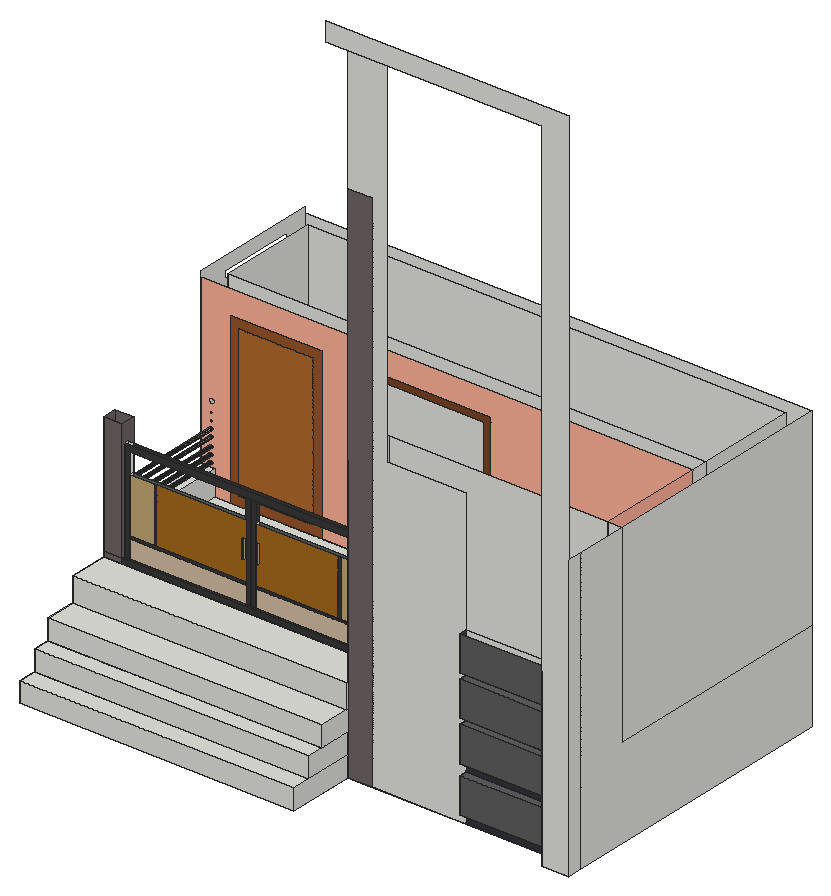
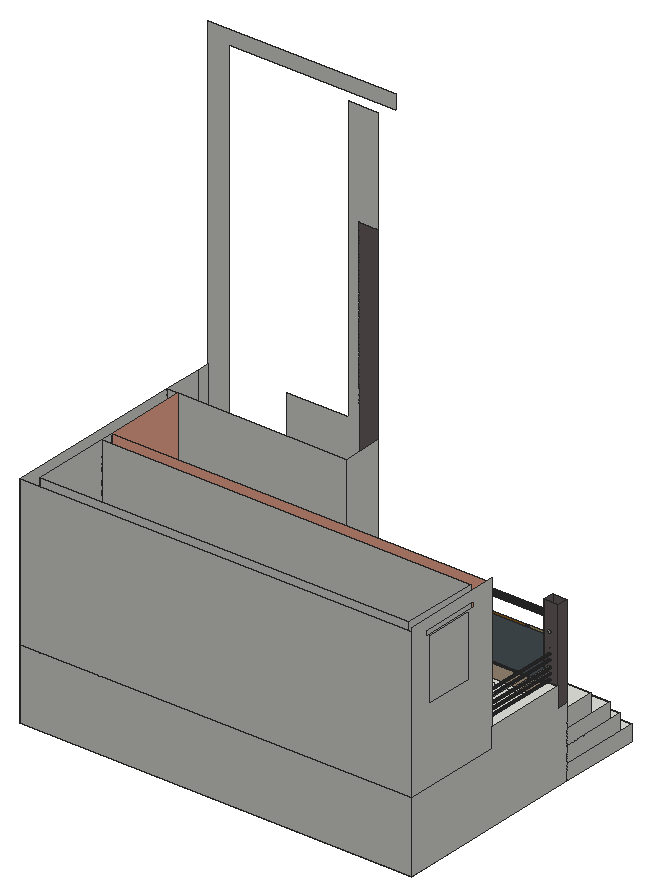
# SketchUp Ruby script. Lengths in inches.
U = 1.inch
M = Sketchup.active_model
def pt(a) = Geom::Point3d.new(a.map { |v| v * U })
def face(e, loops, mat)
  f = e.add_face(loops[0].map { |a| pt(a) })
  loops[1..].each { |l| e.add_face(l.map { |a| pt(a) }).erase! }
  f.material = f.back_material = mat if mat
  f
end
# faces: each face lists its corners as indices into pts; further lists are holes
def faces(e, pts, list, mat = nil) = list.each { |f| face(e, (f[0].is_a?(Array) ? f : [f]).map { |l| l.map { |i| pts[i] } }, mat) }
# xy, xz, yz: faces in a plane at the given z, y or x. An outline is a flat list of corners, or four numbers for a rectangle; further outlines are holes
def ring(l) = l.size == 4 ? [[l[0], l[1]], [l[2], l[1]], [l[2], l[3]], [l[0], l[3]]] : l.each_slice(2).to_a
def flat(e, list, mat, &to3) = list.each { |f| face(e, (f[0].is_a?(Array) ? f : [f]).map { |l| ring(l).map { |u, v| to3.(u, v) } }, mat) }
def xy(e, z, list, mat = nil) = flat(e, list, mat) { |x, y| [x, y, z] }
def xz(e, y, list, mat = nil) = flat(e, list, mat) { |x, z| [x, y, z] }
def yz(e, x, list, mat = nil) = flat(e, list, mat) { |y, z| [x, y, z] }
def lines(e, pts, list) = list.each { |a, b| e.add_line(pt(pts[a]), pt(pts[b])) }
# prism: a flat outline (further loops are holes) pulled along v
def prism(e, loops, v, mat = nil)
  f = face(e, loops, mat); d = Geom::Vector3d.new(v.map { |x| x * U })
  f.pushpull(f.normal.samedirection?(d) ? d.length : -d.length)
end
def box(e, o, s, mat = nil) = prism(e, [[o, [o[0] + s[0], o[1], o[2]], [o[0] + s[0], o[1] + s[1], o[2]], [o[0], o[1] + s[1], o[2]]]], [0, 0, s[2]], mat)
def at(x, y, z, deg = 0) = Geom::Transformation.translation(pt([x, y, z])) * Geom::Transformation.rotation(ORIGIN, Z_AXIS, deg.degrees)
def axes(o, x, y, z) = Geom::Transformation.new([*x, 0, *y, 0, *z, 0, *pt(o).to_a, 1])
def part(name) = M.definitions.add(name)
# library, detail: a bought-in or finely detailed component or shape, given as its bounding box
def library(name, o, s) = part(name).tap { |d| box(d.entities, o, s) }
def detail(e, o, s) = box(e.add_group.entities, o, s)
def put(e, d, t, mat = nil) = e.add_instance(d, t).tap { |i| i.material = mat if mat }
def group(e, t, mat = nil) = e.add_group.tap { |g| g.transformation = t; g.material = mat if mat }.entities
root = M.entities
M.materials.add("[Asphalt New]").color = [112, 100, 103]
M.materials.add("[Blinds Weave]").color = [165, 106, 29]
M.materials.add("[Color B02]").color = [255, 178, 153]
M.materials.add("[Color M07]").color = [58, 58, 58]
M.materials.add("[Formica Beige]").color = [211, 187, 149]
M.materials.add("[Formica Graystone]").color = [149, 146, 135]
M.materials.add("[Formica Laminate Dark]").color = [50, 53, 60]
M.materials.add("[Formica Laminate Light]").color = [213, 189, 164]
M.materials.add("[Formica Speckled Grey]").color = [94, 105, 111]
M.materials.add("[Granite Dark Gray]").color = [96, 95, 95]
M.materials.add("[Granite Dark Gray]1").color = [69, 68, 68]
M.materials.add("[Stone Brushed Khaki]").color = [193, 168, 114]
M.materials.add("[Wood Bamboo]").color = [177, 105, 43]
M.materials.add("[Wood Cherry Original]").color = [152, 86, 42]
M.materials.add("[Wood Veneer 01]").color = [120, 70, 37]
xy(root,0,[[16.8125,0,187.4,65.24],[315.98,32.62,332.57,42.24],[187.4,42.24,187.4,65.24,16.8125,65.24,16.8125,222.09,332.57,222.09,332.57,42.24]])
xy(root,7.28,[[261.19,37.37,316.01,42.24]],"[Granite Dark Gray]")
xy(root,12.75,[[16.8125,0,187.4,11.55],[16.8125,11.55,187.4,65.24]])
xy(root,25.49,[[16.8125,11.55,187.4,21.99],[16.8125,21.99,187.4,65.24]])
xy(root,29.1,[[261.19,37.37,316.01,42.24]],"[Granite Dark Gray]")
xy(root,35.87,[[261.16,37.37,315.98,42.24]],"[Granite Dark Gray]")
xy(root,38.01,[[16.8125,21.99,187.4,41.24],[16.8125,41.24,187.4,65.24]])
xy(root,53.25,[[16.8125,41.24,187.4,65.24]])
xy(root,56.5,[[16.8125,65.24,28.37,74.24],[28.37,67.2,31.31,69.74],[31.31,67.2,103.91,69.74],[103.91,67.2,107.01,69.74],[107.01,67.2,110.1,69.74],
  [110.1,67.2,182.65,69.74],[182.65,67.2,187.4,69.74],[28.37,69.74,187.4,74.24],[323.57,74.24,323.57,213.09,25.8125,213.09,25.8125,140.77,16.8125,140.77,16.8125,222.09,332.57,222.09,332.57,74.24],[25.8125,74.24,323.57,140.77],
  [25.8125,140.77,323.57,150.79],[25.8125,150.79,323.57,213.09]])
xy(root,56.5,[[28.37,65.24,187.4,67.2]],"[Color M07]")
xy(root,57.6875,[[261.16,37.37,315.98,42.24]],"[Granite Dark Gray]")
xy(root,61.24,[[261.16,37.37,315.98,42.24]],"[Granite Dark Gray]")
xy(root,67.27,[[31.31,67.2,103.91,69.74],[110.1,67.2,182.65,69.74]])
xy(root,68.91,[[31.31,67.2,103.91,69.74],[110.1,67.2,182.65,69.74]])
xy(root,72.4375,[[16.8125,74.24,25.8125,140.77]])
xy(root,81.59,[[101.93,66.38,103.24,67.2],[110.62,66.38,111.93,67.2]],"[Formica Beige]")
xy(root,83.0625,[[261.16,37.37,315.98,42.24]],"[Granite Dark Gray]")
xy(root,86.62,[[261.16,37.37,315.98,42.24]],"[Granite Dark Gray]")
xy(root,92.78,[[101.93,66.38,103.24,67.2],[110.62,66.38,111.93,67.2]],"[Formica Beige]")
xz(root,0,[[16.8125,0,187.4,12.75]])
xz(root,11.55,[[16.8125,12.75,187.4,25.49]])
xz(root,21.99,[[16.8125,25.49,187.4,38.01]])
xz(root,32.62,[[315.98,0,332.57,0,332.57,424.6875,181.33,424.6875,181.33,412.9375,315.98,412.9375,315.98,35.87,316.01,29.1,316.01,7.28]])
xz(root,37.37,[[261.19,7.28,316.01,29.1],[261.16,35.87,315.98,57.6875],[261.16,61.24,315.98,83.0625],[261.16,86.62,315.98,108.4375]],"[Granite Dark Gray]")
xz(root,41.24,[[16.8125,38.01,187.4,53.25]])
xz(root,42.24,[[202.71,0,261.16,0,261.19,7.28,261.19,29.1,261.16,35.87,261.16,184.75,211.57,184.75,211.57,412.9375,187.4,412.9375,187.4,328.8125,202.71,328.8125],[261.19,7.28,316.01,29.1],[261.16,35.87,315.98,57.6875],[261.16,61.24,315.98,83.0625],[261.16,86.62,315.98,108.4375]])
xz(root,42.24,[[187.4,0,202.71,328.8125]],"[Asphalt New]")
xz(root,42.24,[[261.16,0,315.98,0,316.01,7.28,261.19,7.28],[261.19,29.1,316.01,29.1,315.98,35.87,261.16,35.87],[261.16,57.6875,315.98,61.24],[261.16,83.0625,315.98,86.62]],"[Formica Laminate Dark]")
xz(root,65.24,[[16.8125,0,187.4,12.75],[16.8125,12.75,187.4,25.49],[16.8125,25.49,187.4,38.01],[16.8125,38.01,187.4,53.25]])
xz(root,65.24,[[16.8125,53.25,28.37,56.5],[16.8125,56.5,28.37,131.3125]],"[Asphalt New]")
xz(root,65.24,[[28.37,53.25,187.4,56.5]],"[Color M07]")
xz(root,66.38,[[101.93,81.59,103.24,92.78],[110.62,81.59,111.93,92.78]],"[Formica Beige]")
xz(root,67.2,[[101.93,81.59,103.24,92.78],[110.62,81.59,111.93,92.78]])
xz(root,67.2,[[[48.18,68.91,103.91,103.37],[101.93,81.59,103.24,92.78]],[[110.1,68.91,160.96,103.37],[110.62,81.59,111.93,92.78]]],"[Blinds Weave]")
xz(root,67.2,[[28.37,56.5,31.31,56.5,31.31,116.1,182.65,116.1,182.65,56.5,187.4,56.5,187.4,119.87,28.37,119.87],[103.91,56.5,107.01,116.1],[107.01,56.5,110.1,116.1],[31.31,67.27,103.91,68.91],[110.1,67.27,182.65,68.91],
  [46.28,68.91,48.18,103.37],[160.96,68.91,162.87,103.37]],"[Color M07]")
xz(root,67.2,[[31.31,56.5,103.91,67.27],[110.1,56.5,182.65,67.27]],"[Formica Laminate Light]")
xz(root,67.2,[[31.31,68.91,46.28,103.37],[162.87,68.91,182.65,103.37]],"[Stone Brushed Khaki]")
xz(root,69.74,[[28.37,56.5,31.31,119.87]])
xz(root,69.74,[[182.65,56.5,182.65,116.1,31.31,116.1,31.31,119.87,187.4,119.87,187.4,56.5],[103.91,56.5,107.01,116.1],[107.01,56.5,110.1,116.1],[31.31,67.27,103.91,68.91],[110.1,67.27,182.65,68.91]],"[Color M07]")
xz(root,69.74,[[31.31,56.5,103.91,67.27],[110.1,56.5,182.65,67.27]],"[Formica Laminate Light]")
xz(root,69.74,[[31.31,68.91,103.91,103.37],[110.1,68.91,182.65,103.37]],"[Formica Speckled Grey]")
xz(root,74.24,[[16.8125,56.5,25.8125,72.4375],[187.4,56.5,323.57,176.5],[323.57,56.5,332.57,176.5],[23.42,74.0625,23.65,74.09,23.86,74.18,24.04,74.32,24.18,74.5,24.27,74.71,24.3,74.9375,24.27,75.16,24.18,75.375,24.04,75.56,23.86,75.69,23.65,75.78,23.42,75.8125,23.2,75.78,22.99,75.69,22.81,75.56,22.67,75.375,22.58,75.16,22.55,74.9375,22.58,74.71,22.67,74.5,22.81,74.32,22.99,74.18,23.2,74.09],[23.42,78.5625,23.65,78.59,23.86,78.68,24.04,78.82,24.18,79,24.27,79.21,24.3,79.4375,24.27,79.66,24.18,79.875,24.04,80.06,23.86,80.19,23.65,80.28,23.42,80.3125,23.2,80.28,22.99,80.19,22.81,80.06,22.67,79.875,22.58,79.66,22.55,79.4375,22.58,79.21,22.67,79,22.81,78.82,22.99,78.68,23.2,78.59],
  [23.42,82.9375,23.65,82.97,23.86,83.05,24.04,83.19,24.18,83.375,24.27,83.59,24.3,83.8125,24.27,84.04,24.18,84.25,24.04,84.43,23.86,84.57,23.65,84.66,23.42,84.6875,23.2,84.66,22.99,84.57,22.81,84.43,22.67,84.25,22.58,84.04,22.55,83.8125,22.58,83.59,22.67,83.375,22.81,83.19,22.99,83.05,23.2,82.97],[23.42,88.375,23.65,88.4,23.86,88.49,24.04,88.63,24.18,88.8125,24.27,89.02,24.3,89.25,24.27,89.48,24.18,89.6875,24.04,89.87,23.86,90.01,23.65,90.09,23.42,90.125,23.2,90.09,22.99,90.01,22.81,89.87,22.67,89.6875,22.58,89.48,22.55,89.25,22.58,89.02,22.67,88.8125,22.81,88.63,22.99,88.49,23.2,88.4],[23.42,92.875,23.65,92.9,23.86,92.99,24.04,93.13,24.18,93.3125,24.27,93.52,24.3,93.75,24.27,93.98,24.18,94.1875,24.04,94.37,23.86,94.51,23.65,94.59,23.42,94.625,23.2,94.59,22.99,94.51,22.81,94.37,22.67,94.1875,22.58,93.98,22.55,93.75,22.58,93.52,22.67,93.3125,22.81,93.13,22.99,92.99,23.2,92.9]])
xz(root,74.24,[[[25.8125,56.5,25.8125,72.4375,16.8125,72.4375,16.8125,131.3125,28.37,131.3125,28.37,56.5],[23.64,107.65,24.1,107.71,24.54,107.89,24.92,108.18,25.2,108.56,25.39,109,25.45,109.46,25.39,109.93,25.2,110.37,24.92,110.75,24.54,111.03,24.1,111.21,23.64,111.28,23.17,111.21,22.73,111.03,22.35,110.75,22.07,110.37,21.88,109.93,21.82,109.46,21.88,109,22.07,108.56,22.35,108.18,22.73,107.89,23.17,107.71],[23.42,74.0625,23.65,74.09,23.86,74.18,24.04,74.32,24.18,74.5,24.27,74.71,24.3,74.9375,24.27,75.16,24.18,75.375,24.04,75.56,23.86,75.69,23.65,75.78,23.42,75.8125,23.2,75.78,22.99,75.69,22.81,75.56,22.67,75.375,22.58,75.16,22.55,74.9375,22.58,74.71,22.67,74.5,22.81,74.32,22.99,74.18,23.2,74.09],[23.42,97.3125,23.65,97.34,23.86,97.43,24.04,97.57,24.18,97.75,24.27,97.96,24.3,98.1875,24.27,98.41,24.18,98.625,24.04,98.81,23.86,98.94,23.65,99.03,23.42,99.0625,23.2,99.03,22.99,98.94,22.81,98.81,22.67,98.625,22.58,98.41,22.55,98.1875,22.58,97.96,22.67,97.75,22.81,97.57,22.99,97.43,23.2,97.34],[23.42,78.5625,23.65,78.59,23.86,78.68,24.04,78.82,24.18,79,24.27,79.21,24.3,79.4375,24.27,79.66,24.18,79.875,24.04,80.06,23.86,80.19,23.65,80.28,23.42,80.3125,23.2,80.28,22.99,80.19,22.81,80.06,22.67,79.875,22.58,79.66,22.55,79.4375,22.58,79.21,22.67,79,22.81,78.82,22.99,78.68,23.2,78.59],[23.42,92.875,23.65,92.9,23.86,92.99,24.04,93.13,24.18,93.3125,24.27,93.52,24.3,93.75,24.27,93.98,24.18,94.1875,24.04,94.37,23.86,94.51,23.65,94.59,23.42,94.625,23.2,94.59,22.99,94.51,22.81,94.37,22.67,94.1875,22.58,93.98,22.55,93.75,22.58,93.52,22.67,93.3125,22.81,93.13,22.99,92.99,23.2,92.9],[23.42,82.9375,23.65,82.97,23.86,83.05,24.04,83.19,24.18,83.375,24.27,83.59,24.3,83.8125,24.27,84.04,24.18,84.25,24.04,84.43,23.86,84.57,23.65,84.66,23.42,84.6875,23.2,84.66,22.99,84.57,22.81,84.43,22.67,84.25,22.58,84.04,22.55,83.8125,22.58,83.59,22.67,83.375,22.81,83.19,22.99,83.05,23.2,82.97],[23.42,88.375,23.65,88.4,23.86,88.49,24.04,88.63,24.18,88.8125,24.27,89.02,24.3,89.25,24.27,89.48,24.18,89.6875,24.04,89.87,23.86,90.01,23.65,90.09,23.42,90.125,23.2,90.09,22.99,90.01,22.81,89.87,22.67,89.6875,22.58,89.48,22.55,89.25,22.58,89.02,22.67,88.8125,22.81,88.63,22.99,88.49,23.2,88.4],[23.42,101.875,23.65,101.9,23.86,101.99,24.04,102.13,24.18,102.3125,24.27,102.52,24.3,102.75,24.27,102.98,24.18,103.1875,24.04,103.37,23.86,103.51,23.65,103.59,23.42,103.625,23.2,103.59,22.99,103.51,22.81,103.37,22.67,103.1875,22.58,102.98,22.55,102.75,22.58,102.52,22.67,102.3125,22.81,102.13,22.99,101.99,23.2,101.9]]],"[Asphalt New]")
xz(root,140.77,[[16.8125,56.5,25.8125,72.4375]])
xz(root,140.77,[[[25.8125,56.5,34.96,56.5,34.96,161.375,92.77,161.375,92.77,56.5,323.57,56.5,323.57,176.5,16.8125,176.5,16.8125,72.4375,25.8125,72.4375],[113.52,94.78,197.34,161.41],[23.64,107.65,23.17,107.71,22.73,107.89,22.35,108.18,22.07,108.56,21.88,109,21.82,109.46,21.88,109.93,22.07,110.37,22.35,110.75,22.73,111.03,23.17,111.21,23.64,111.28,24.1,111.21,24.54,111.03,24.92,110.75,25.2,110.37,25.39,109.93,25.45,109.46,25.39,109,25.2,108.56,24.92,108.18,24.54,107.89,24.1,107.71],[23.42,82.9375,23.2,82.97,22.99,83.05,22.81,83.19,22.67,83.375,22.58,83.59,22.55,83.8125,22.58,84.04,22.67,84.25,22.81,84.43,22.99,84.57,23.2,84.66,23.42,84.6875,23.65,84.66,23.86,84.57,24.04,84.43,24.18,84.25,24.27,84.04,24.3,83.8125,24.27,83.59,24.18,83.375,24.04,83.19,23.86,83.05,23.65,82.97],[23.42,78.5625,23.2,78.59,22.99,78.68,22.81,78.82,22.67,79,22.58,79.21,22.55,79.4375,22.58,79.66,22.67,79.875,22.81,80.06,22.99,80.19,23.2,80.28,23.42,80.3125,23.65,80.28,23.86,80.19,24.04,80.06,24.18,79.875,24.27,79.66,24.3,79.4375,24.27,79.21,24.18,79,24.04,78.82,23.86,78.68,23.65,78.59],[23.42,74.0625,23.2,74.09,22.99,74.18,22.81,74.32,22.67,74.5,22.58,74.71,22.55,74.9375,22.58,75.16,22.67,75.375,22.81,75.56,22.99,75.69,23.2,75.78,23.42,75.8125,23.65,75.78,23.86,75.69,24.04,75.56,24.18,75.375,24.27,75.16,24.3,74.9375,24.27,74.71,24.18,74.5,24.04,74.32,23.86,74.18,23.65,74.09],[23.42,88.375,23.2,88.4,22.99,88.49,22.81,88.63,22.67,88.8125,22.58,89.02,22.55,89.25,22.58,89.48,22.67,89.6875,22.81,89.87,22.99,90.01,23.2,90.09,23.42,90.125,23.65,90.09,23.86,90.01,24.04,89.87,24.18,89.6875,24.27,89.48,24.3,89.25,24.27,89.02,24.18,88.8125,24.04,88.63,23.86,88.49,23.65,88.4],[23.42,92.875,23.2,92.9,22.99,92.99,22.81,93.13,22.67,93.3125,22.58,93.52,22.55,93.75,22.58,93.98,22.67,94.1875,22.81,94.37,22.99,94.51,23.2,94.59,23.42,94.625,23.65,94.59,23.86,94.51,24.04,94.37,24.18,94.1875,24.27,93.98,24.3,93.75,24.27,93.52,24.18,93.3125,24.04,93.13,23.86,92.99,23.65,92.9],[23.42,97.3125,23.2,97.34,22.99,97.43,22.81,97.57,22.67,97.75,22.58,97.96,22.55,98.1875,22.58,98.41,22.67,98.625,22.81,98.81,22.99,98.94,23.2,99.03,23.42,99.0625,23.65,99.03,23.86,98.94,24.04,98.81,24.18,98.625,24.27,98.41,24.3,98.1875,24.27,97.96,24.18,97.75,24.04,97.57,23.86,97.43,23.65,97.34],[23.42,101.875,23.2,101.9,22.99,101.99,22.81,102.13,22.67,102.3125,22.58,102.52,22.55,102.75,22.58,102.98,22.67,103.1875,22.81,103.37,22.99,103.51,23.2,103.59,23.42,103.625,23.65,103.59,23.86,103.51,24.04,103.37,24.18,103.1875,24.27,102.98,24.3,102.75,24.27,102.52,24.18,102.3125,24.04,102.13,23.86,101.99,23.65,101.9]]],"[Color B02]")
xz(root,140.77,[[40.87,62.4,86.87,155.47]],"[Wood Bamboo]")
xz(root,140.77,[[[34.96,56.5,92.77,161.375],[40.87,62.4,86.87,155.47]]],"[Wood Cherry Original]")
xz(root,140.77,[[[113.52,94.78,197.34,161.41],[117.625,98.88,193.24,157.31]]],"[Wood Veneer 01]")
xz(root,150.79,[[25.8125,56.5,323.57,176.5]])
xz(root,213.09,[[25.8125,56.5,323.57,176.5]])
xz(root,222.09,[[16.8125,0,332.57,56.5],[16.8125,56.5,332.57,176.5]])
yz(root,16.8125,[[0,0,65.24,12.75],[65.24,0,65.24,56.5,74.24,56.5,74.24,72.4375,140.77,72.4375,140.77,56.5,222.09,56.5,222.09,0],[11.55,12.75,65.24,25.49],[21.99,25.49,65.24,38.01],[41.24,38.01,65.24,53.25],
  [[140.77,56.5,222.09,179.875],[163.89,116.83,204.58,166.46],[159.31,167.09,207.81,171.34]]])
yz(root,16.8125,[[65.24,56.5,74.24,131.3125]],"[Asphalt New]")
yz(root,25.8125,[[74.24,56.5,140.77,72.4375],[150.79,56.5,213.09,176.5]])
yz(root,28.37,[[67.2,56.5,69.74,119.87]])
yz(root,28.37,[[65.24,56.5,67.2,56.5,67.2,119.87,69.74,119.87,69.74,56.5,74.24,56.5,74.24,131.3125,65.24,131.3125]],"[Asphalt New]")
yz(root,31.31,[[67.2,56.5,69.74,67.27],[67.2,67.27,69.74,68.91],[67.2,68.91,69.74,103.37]])
yz(root,101.93,[[66.38,81.59,67.2,92.78]],"[Formica Beige]")
yz(root,103.24,[[66.38,81.59,67.2,92.78]],"[Formica Beige]")
yz(root,103.91,[[67.2,67.27,69.74,68.91]])
yz(root,107.01,[[67.2,56.5,69.74,116.1]])
yz(root,110.1,[[67.2,56.5,69.74,67.27],[67.2,67.27,69.74,68.91],[67.2,68.91,69.74,103.37]])
yz(root,110.62,[[66.38,81.59,67.2,92.78]],"[Formica Beige]")
yz(root,111.93,[[66.38,81.59,67.2,92.78]],"[Formica Beige]")
yz(root,182.65,[[67.2,67.27,69.74,68.91]])
yz(root,187.4,[[0,0,42.24,12.75],[42.24,0,65.24,12.75],[11.55,12.75,42.24,25.49],[42.24,12.75,65.24,25.49],[21.99,25.49,42.24,38.01],
  [42.24,25.49,65.24,38.01],[41.24,38.01,42.24,53.25],[42.24,38.01,65.24,53.25],[42.24,53.25,42.24,176.5,74.24,176.5,74.24,56.5,69.74,56.5,69.74,119.87,67.2,119.87,67.2,56.5,65.24,56.5,65.24,53.25],[67.2,56.5,69.74,119.87]])
yz(root,261.16,[[37.37,35.87,42.24,57.6875],[37.37,61.24,42.24,83.0625],[37.37,86.62,42.24,108.4375]],"[Granite Dark Gray]1")
yz(root,261.19,[[37.37,7.28,42.24,29.1]],"[Granite Dark Gray]1")
yz(root,315.98,[[32.62,35.87,37.37,57.6875],[37.37,35.87,42.24,57.6875],[32.62,57.6875,42.24,61.24],[32.62,61.24,37.37,83.0625],[37.37,61.24,42.24,83.0625],
  [32.62,83.0625,42.24,86.62],[32.62,86.62,37.37,108.4375],[37.37,86.62,42.24,108.4375]])
yz(root,316.01,[[32.62,7.28,37.37,29.1],[37.37,7.28,42.24,29.1]])
yz(root,323.57,[[140.77,56.5,150.79,176.5],[150.79,56.5,213.09,176.5]])
yz(root,323.57,[[74.24,56.5,140.77,176.5]],"[Color B02]")
yz(root,332.57,[[32.62,0,42.24,176.5],[42.24,0,222.09,0,222.09,56.5,74.24,56.5,74.24,176.5,42.24,176.5],[74.24,56.5,222.09,176.5]])
p = [[316.01,42.24,7.28],[315.98,42.24,0],[315.98,32.62,0],[316.01,32.62,7.28],[316.01,37.37,7.28],[315.98,42.24,35.87],
  [316.01,42.24,29.1],[316.01,37.37,29.1],[316.01,32.62,29.1],[315.98,32.62,35.87],[315.98,37.37,35.87],[23.2,74.24,74.09],
  [22.99,74.24,74.18],[22.99,140.77,74.18],[23.2,140.77,74.09],[23.42,74.24,74.0625],[23.42,140.77,74.0625],[23.65,74.24,74.09],
  [23.65,140.77,74.09],[23.86,74.24,74.18],[23.86,140.77,74.18],[22.81,74.24,74.32],[22.81,140.77,74.32],[24.04,74.24,74.32],
  [24.04,140.77,74.32],[22.67,74.24,74.5],[22.67,140.77,74.5],[24.18,74.24,74.5],[24.18,140.77,74.5],[22.58,74.24,74.71],
  [22.58,140.77,74.71],[24.27,74.24,74.71],[24.27,140.77,74.71],[22.55,74.24,74.9375],[22.55,140.77,74.9375],[24.3,74.24,74.9375],
  [24.3,140.77,74.9375],[22.58,74.24,75.16],[22.58,140.77,75.16],[24.27,74.24,75.16],[24.27,140.77,75.16],[22.67,74.24,75.375],
  [22.67,140.77,75.375],[24.18,74.24,75.375],[24.18,140.77,75.375],[22.81,74.24,75.56],[22.81,140.77,75.56],[24.04,74.24,75.56],
  [24.04,140.77,75.56],[22.99,74.24,75.69],[22.99,140.77,75.69],[23.86,74.24,75.69],[23.86,140.77,75.69],[23.2,74.24,75.78],
  [23.2,140.77,75.78],[23.65,74.24,75.78],[23.65,140.77,75.78],[23.42,74.24,75.8125],[23.42,140.77,75.8125],[23.2,74.24,78.59],
  [22.99,74.24,78.68],[22.99,140.77,78.68],[23.2,140.77,78.59],[23.42,74.24,78.5625],[23.42,140.77,78.5625],[23.65,74.24,78.59],
  [23.65,140.77,78.59],[23.86,74.24,78.68],[23.86,140.77,78.68],[22.81,74.24,78.82],[22.81,140.77,78.82],[24.04,74.24,78.82],
  [24.04,140.77,78.82],[22.67,74.24,79],[22.67,140.77,79],[24.18,74.24,79],[24.18,140.77,79],[22.58,74.24,79.21],
  [22.58,140.77,79.21],[24.27,74.24,79.21],[24.27,140.77,79.21],[22.55,74.24,79.4375],[22.55,140.77,79.4375],[24.3,74.24,79.4375],
  [24.3,140.77,79.4375],[22.58,74.24,79.66],[22.58,140.77,79.66],[24.27,74.24,79.66],[24.27,140.77,79.66],[22.67,74.24,79.875],
  [22.67,140.77,79.875],[24.18,74.24,79.875],[24.18,140.77,79.875],[22.81,74.24,80.06],[22.81,140.77,80.06],[24.04,74.24,80.06],
  [24.04,140.77,80.06],[22.99,74.24,80.19],[22.99,140.77,80.19],[23.86,74.24,80.19],[23.86,140.77,80.19],[23.2,74.24,80.28],
  [23.2,140.77,80.28],[23.65,74.24,80.28],[23.65,140.77,80.28],[23.42,74.24,80.3125],[23.42,140.77,80.3125],[23.42,74.24,82.9375],
  [23.2,74.24,82.97],[23.2,140.77,82.97],[23.42,140.77,82.9375],[23.65,74.24,82.97],[23.65,140.77,82.97],[22.99,74.24,83.05],
  [22.99,140.77,83.05],[23.86,74.24,83.05],[23.86,140.77,83.05],[22.81,74.24,83.19],[22.81,140.77,83.19],[24.04,74.24,83.19],
  [24.04,140.77,83.19],[22.67,74.24,83.375],[22.67,140.77,83.375],[24.18,74.24,83.375],[24.18,140.77,83.375],[22.58,74.24,83.59],
  [22.58,140.77,83.59],[24.27,74.24,83.59],[24.27,140.77,83.59],[22.55,74.24,83.8125],[22.55,140.77,83.8125],[24.3,74.24,83.8125],
  [24.3,140.77,83.8125],[22.58,74.24,84.04],[22.58,140.77,84.04],[24.27,74.24,84.04],[24.27,140.77,84.04],[22.67,74.24,84.25],
  [22.67,140.77,84.25],[24.18,74.24,84.25],[24.18,140.77,84.25],[22.81,74.24,84.43],[22.81,140.77,84.43],[24.04,74.24,84.43],
  [24.04,140.77,84.43],[22.99,74.24,84.57],[22.99,140.77,84.57],[23.86,74.24,84.57],[23.86,140.77,84.57],[23.2,74.24,84.66],
  [23.2,140.77,84.66],[23.65,74.24,84.66],[23.65,140.77,84.66],[23.42,74.24,84.6875],[23.42,140.77,84.6875],[23.2,74.24,88.4],
  [22.99,74.24,88.49],[22.99,140.77,88.49],[23.2,140.77,88.4],[23.42,74.24,88.375],[23.42,140.77,88.375],[23.65,74.24,88.4],
  [23.65,140.77,88.4],[23.86,74.24,88.49],[23.86,140.77,88.49],[22.81,74.24,88.63],[22.81,140.77,88.63],[24.04,74.24,88.63],
  [24.04,140.77,88.63],[22.67,74.24,88.8125],[22.67,140.77,88.8125],[24.18,74.24,88.8125],[24.18,140.77,88.8125],[22.58,74.24,89.02],
  [22.58,140.77,89.02],[24.27,74.24,89.02],[24.27,140.77,89.02],[22.55,74.24,89.25],[22.55,140.77,89.25],[24.3,74.24,89.25],
  [24.3,140.77,89.25],[22.58,74.24,89.48],[22.58,140.77,89.48],[24.27,74.24,89.48],[24.27,140.77,89.48],[22.67,74.24,89.6875],
  [22.67,140.77,89.6875],[24.18,74.24,89.6875],[24.18,140.77,89.6875],[22.81,74.24,89.87],[22.81,140.77,89.87],[24.04,74.24,89.87],
  [24.04,140.77,89.87],[22.99,74.24,90.01],[22.99,140.77,90.01],[23.86,74.24,90.01],[23.86,140.77,90.01],[23.2,74.24,90.09],
  [23.2,140.77,90.09],[23.65,74.24,90.09],[23.65,140.77,90.09],[23.42,74.24,90.125],[23.42,140.77,90.125],[23.2,74.24,92.9],
  [22.99,74.24,92.99],[22.99,140.77,92.99],[23.2,140.77,92.9],[23.42,74.24,92.875],[23.42,140.77,92.875],[23.65,74.24,92.9],
  [23.65,140.77,92.9],[23.86,74.24,92.99],[23.86,140.77,92.99],[22.81,74.24,93.13],[22.81,140.77,93.13],[24.04,74.24,93.13],
  [24.04,140.77,93.13],[22.67,74.24,93.3125],[22.67,140.77,93.3125],[24.18,74.24,93.3125],[24.18,140.77,93.3125],[22.58,74.24,93.52],
  [22.58,140.77,93.52],[24.27,74.24,93.52],[24.27,140.77,93.52],[22.55,74.24,93.75],[22.55,140.77,93.75],[24.3,74.24,93.75],
  [24.3,140.77,93.75],[22.58,74.24,93.98],[22.58,140.77,93.98],[24.27,74.24,93.98],[24.27,140.77,93.98],[22.67,74.24,94.1875],
  [22.67,140.77,94.1875],[24.18,74.24,94.1875],[24.18,140.77,94.1875],[22.81,74.24,94.37],[22.81,140.77,94.37],[24.04,74.24,94.37],
  [24.04,140.77,94.37],[22.99,74.24,94.51],[22.99,140.77,94.51],[23.86,74.24,94.51],[23.86,140.77,94.51],[23.2,74.24,94.59],
  [23.2,140.77,94.59],[23.65,74.24,94.59],[23.65,140.77,94.59],[23.42,74.24,94.625],[23.42,140.77,94.625]]
faces(root,p,[[0,1,2,3,4],[5,6,7,8,9,10]])
faces(root,p,[[11,12,13,14],[15,11,14,16],[17,15,16,18],[19,17,18,20],[12,21,22,13],[23,19,20,24],[21,25,26,22],[27,23,24,28],
  [25,29,30,26],[31,27,28,32],[29,33,34,30],[35,31,32,36],[33,37,38,34],[39,35,36,40],[37,41,42,38],[43,39,40,44],
  [41,45,46,42],[47,43,44,48],[45,49,50,46],[51,47,48,52],[49,53,54,50],[55,51,52,56],[53,57,58,54],[57,55,56,58],
  [59,60,61,62],[63,59,62,64],[65,63,64,66],[67,65,66,68],[60,69,70,61],[71,67,68,72],[69,73,74,70],[75,71,72,76],
  [73,77,78,74],[79,75,76,80],[77,81,82,78],[83,79,80,84],[81,85,86,82],[87,83,84,88],[85,89,90,86],[91,87,88,92],
  [89,93,94,90],[95,91,92,96],[93,97,98,94],[99,95,96,100],[97,101,102,98],[103,99,100,104],[101,105,106,102],[105,103,104,106],
  [107,108,109,110],[111,107,110,112],[108,113,114,109],[115,111,112,116],[113,117,118,114],[119,115,116,120],[117,121,122,118],[123,119,120,124],
  [121,125,126,122],[127,123,124,128],[125,129,130,126],[131,127,128,132],[129,133,134,130],[135,131,132,136],[133,137,138,134],[139,135,136,140],
  [137,141,142,138],[143,139,140,144],[141,145,146,142],[147,143,144,148],[145,149,150,146],[151,147,148,152],[149,153,154,150],[153,151,152,154],
  [155,156,157,158],[159,155,158,160],[161,159,160,162],[163,161,162,164],[156,165,166,157],[167,163,164,168],[165,169,170,166],[171,167,168,172],
  [169,173,174,170],[175,171,172,176],[173,177,178,174],[179,175,176,180],[177,181,182,178],[183,179,180,184],[181,185,186,182],[187,183,184,188],
  [185,189,190,186],[191,187,188,192],[189,193,194,190],[195,191,192,196],[193,197,198,194],[199,195,196,200],[197,201,202,198],[201,199,200,202],
  [203,204,205,206],[207,203,206,208],[209,207,208,210],[211,209,210,212],[204,213,214,205],[215,211,212,216],[213,217,218,214],[219,215,216,220],
  [217,221,222,218],[223,219,220,224],[221,225,226,222],[227,223,224,228],[225,229,230,226],[231,227,228,232],[229,233,234,230],[235,231,232,236],
  [233,237,238,234],[239,235,236,240],[237,241,242,238],[243,239,240,244],[241,245,246,242],[247,243,244,248],[245,249,250,246],[249,247,248,250]],"[Formica Graystone]")
